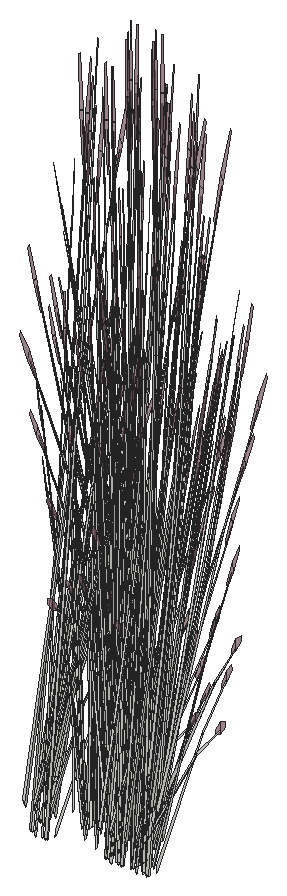
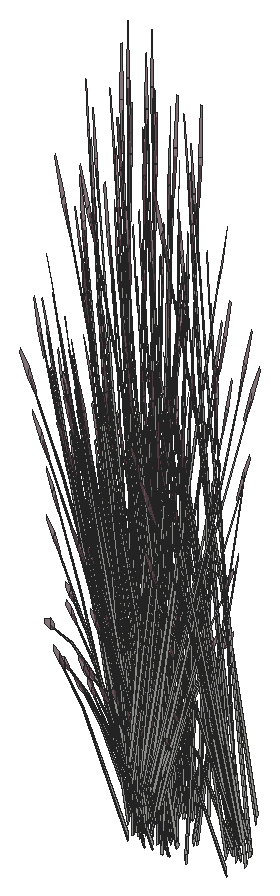
# SketchUp Ruby script. Lengths in inches.
U = 1.inch
M = Sketchup.active_model
def pt(a) = Geom::Point3d.new(a.map { |v| v * U })
def face(e, loops, mat)
  f = e.add_face(loops[0].map { |a| pt(a) })
  loops[1..].each { |l| e.add_face(l.map { |a| pt(a) }).erase! }
  f.material = f.back_material = mat if mat
  f
end
# faces: each face lists its corners as indices into pts; further lists are holes
def faces(e, pts, list, mat = nil) = list.each { |f| face(e, (f[0].is_a?(Array) ? f : [f]).map { |l| l.map { |i| pts[i] } }, mat) }
# xy, xz, yz: faces in a plane at the given z, y or x. An outline is a flat list of corners, or four numbers for a rectangle; further outlines are holes
def ring(l) = l.size == 4 ? [[l[0], l[1]], [l[2], l[1]], [l[2], l[3]], [l[0], l[3]]] : l.each_slice(2).to_a
def flat(e, list, mat, &to3) = list.each { |f| face(e, (f[0].is_a?(Array) ? f : [f]).map { |l| ring(l).map { |u, v| to3.(u, v) } }, mat) }
def xy(e, z, list, mat = nil) = flat(e, list, mat) { |x, y| [x, y, z] }
def xz(e, y, list, mat = nil) = flat(e, list, mat) { |x, z| [x, y, z] }
def yz(e, x, list, mat = nil) = flat(e, list, mat) { |y, z| [x, y, z] }
def lines(e, pts, list) = list.each { |a, b| e.add_line(pt(pts[a]), pt(pts[b])) }
# prism: a flat outline (further loops are holes) pulled along v
def prism(e, loops, v, mat = nil)
  f = face(e, loops, mat); d = Geom::Vector3d.new(v.map { |x| x * U })
  f.pushpull(f.normal.samedirection?(d) ? d.length : -d.length)
end
def box(e, o, s, mat = nil) = prism(e, [[o, [o[0] + s[0], o[1], o[2]], [o[0] + s[0], o[1] + s[1], o[2]], [o[0], o[1] + s[1], o[2]]]], [0, 0, s[2]], mat)
def at(x, y, z, deg = 0) = Geom::Transformation.translation(pt([x, y, z])) * Geom::Transformation.rotation(ORIGIN, Z_AXIS, deg.degrees)
def axes(o, x, y, z) = Geom::Transformation.new([*x, 0, *y, 0, *z, 0, *pt(o).to_a, 1])
def part(name) = M.definitions.add(name)
# library, detail: a bought-in or finely detailed component or shape, given as its bounding box
def library(name, o, s) = part(name).tap { |d| box(d.entities, o, s) }
def detail(e, o, s) = box(e.add_group.entities, o, s)
def put(e, d, t, mat = nil) = e.add_instance(d, t).tap { |i| i.material = mat if mat }
def group(e, t, mat = nil) = e.add_group.tap { |g| g.transformation = t; g.material = mat if mat }.entities
root = M.entities
M.materials.add("LightPink_Translucent").color = [144, 107, 117]
M.materials["LightPink_Translucent"].alpha = 0.75
c1 = part("blade")
p = [[2.15,0.21,22],[0,0.17,0],[0.09,0.45,0],[2.18,0.31,22],[2.29,0.31,22],[0.38,0.45,0],
  [2.48,0.24,33],[2.49,0.24,33],[2.48,0.22,33]]
faces(c1.entities,p,[[0,1,2,3],[4,5,2,3],[6,3,4,7],[8,0,3,6]])
c2 = part("seeds")
p = [[0.3,-0.1,1.38],[-0.01,-0.03,1.59],[-0.01,-0.03,0.03],[0.14,-0.07,-0.07],[0.29,-0.03,3],[0.15,0.01,3.11]]
faces(c2.entities,p,[[0,1,2,3],[1,0,4,5]],"LightPink_Translucent")
c3 = part("blade with seeds")
put(c3.entities,c1,at(0,0,0))
put(c3.entities,c2,axes([2.4,0.25,30.99],[1.5799,-0.05474,1.17369],[-0.12525,1.92788,0.29478],[-0.07173,-0.02425,1.56792]))
put(root,c3,axes([361.61,660.92,628.08],[0.3879,0.02311,-0.13498],[-0.0106,0.43749,-0.74919],[-0.02694,0.1685,1.13838]))
put(root,c3,axes([360.375,663.42,620.59],[-0.085,-0.1147,1.43002],[0.1106,-0.37943,-0.30754],[0.17198,0.0514,0.61141]))
put(root,c3,axes([362.33,661.41,627.71],[0.34538,-0.21713,-0.1216],[0.16972,0.38536,-0.67495],[0.04557,0.16239,1.02557]))
put(root,c3,axes([362.43,661.56,627.74],[-0.34777,-0.12192,0.53283],[0.11892,-0.40083,0.43934],[0.0209,0.15763,1.10256]))
put(root,c3,axes([361.79,662.16,625.45],[-0.00913,-0.2773,1.1486],[0.22824,0.19778,0.84392],[-0.04489,0.13217,0.25299]))
put(root,c3,axes([356.73,663.82,620.2],[0.35581,0.20937,0],[-0.17124,0.43505,0],[0,0,1.74954]))
put(root,c3,axes([358.86,663.83,620.2],[0.35581,0.20937,0],[-0.17124,0.43505,0],[0,0,1.74954]))
put(root,c3,axes([362.39,661.5,624.17],[0.05712,-0.02538,1.76342],[0.34359,0.13968,-0.26939],[0.01005,0.15742,0.30037]))
put(root,c3,axes([351.3,663.33,622.98],[0.35281,0.01123,-0.71045],[-0.0237,0.47284,0.08574],[0.14947,0.0499,1.00501]))
put(root,c3,axes([357.76,663.58,622.72],[0.07571,-0.00789,1.74944],[0.20767,-0.36231,-0.27667],[0.13467,0.04783,0.14031]))
put(root,c3,axes([356.87,664.28,620.19],[-0.21791,-0.46895,-0.05142],[0.36918,-0.26061,0.51607],[-0.09097,0.04465,1.6363]))
put(root,c3,axes([359.89,663.59,622.72],[0.07571,-0.00789,1.74944],[0.20767,-0.36231,-0.27667],[0.13467,0.04783,0.14031]))
put(root,c3,axes([359,664.3,620.19],[-0.21791,-0.46895,-0.05142],[0.36918,-0.26061,0.51607],[-0.09097,0.04465,1.6363]))
put(root,c3,axes([356.79,663.15,620.62],[0.26075,0.2802,0.1448],[-0.2175,0.31612,-0.41347],[-0.06054,0.04274,1.26744]))
put(root,c3,axes([358.92,663.16,620.62],[0.26075,0.2802,0.1448],[-0.2175,0.31612,-0.41347],[-0.06054,0.04274,1.26744]))
put(root,c3,axes([354.73,663.22,622.73],[-0.08753,-0.42921,0.48003],[0.34336,-0.07449,0.3958],[-0.1012,0.10094,0.9933]))
put(root,c3,axes([356.86,663.24,622.73],[-0.08753,-0.42921,0.48003],[0.34336,-0.07449,0.3958],[-0.1012,0.10094,0.9933]))
put(root,c3,axes([354.67,663.14,622.73],[-0.2423,-0.19613,0.0643],[0.14107,-0.2793,0.50621],[-0.07768,0.0903,0.77189]))
put(root,c3,axes([354.78,662.62,621.875],[0.12246,-0.09864,1.71376],[0.1031,0.45582,0.13857],[-0.19225,0.10302,0.73262]))
put(root,c3,axes([356.79,663.15,622.73],[-0.2423,-0.19613,0.0643],[0.14107,-0.2793,0.50621],[-0.07768,0.0903,0.77189]))
put(root,c3,axes([356.9,662.64,621.875],[0.12246,-0.09864,1.71376],[0.1031,0.45582,0.13857],[-0.19225,0.10302,0.73262]))
put(root,c3,axes([361.875,661.09,627.6875],[0.25266,0.31335,-0.5672],[-0.2669,0.27442,-0.43934],[-0.03844,0.15921,1.08528]))
put(root,c3,axes([361.6,661.56,625.5],[0.32063,-0.08258,0.06507],[0.07371,0.33271,-0.86304],[-0.02033,0.16842,0.7736]))
put(root,c3,axes([362.62,661.39,627.36],[0.34695,0.11691,-0.51099],[-0.11892,0.40083,-0.3958],[0.03181,0.16138,0.97773]))
put(root,c3,axes([362.82,660.57,626.56],[-0.08068,-0.14973,1.71376],[0.3728,-0.12606,0.13857],[0.08426,0.23506,0.73262]))
put(root,c3,axes([351.88,662.37,620.375],[0.44133,0,0],[0,0.52122,-0.51607],[0,0.11871,1.63711]))
put(root,c3,axes([357.47,663.63,622.98],[0.35281,0.01123,-0.71045],[-0.0237,0.47284,0.08574],[0.14947,0.0499,1.00501]))
put(root,c3,axes([359.6,663.65,622.98],[0.35281,0.01123,-0.71045],[-0.0237,0.47284,0.08574],[0.14947,0.0499,1.00501]))
put(root,c3,axes([350.75,662.1875,620.67],[0.39748,0.22252,-0.29095],[-0.19139,0.46966,-0.50002],[0.01249,0.11531,1.59708]))
put(root,c3,axes([357.07,664.01,620.48],[0.33032,-0.23318,0.49651],[0.19744,0.41812,0],[-0.07523,0.05311,1.57504]))
put(root,c3,axes([359.2,664.03,620.48],[0.33032,-0.23318,0.49651],[0.19744,0.41812,0],[-0.07523,0.05311,1.57504]))
put(root,c3,axes([362.46,661.64,627.21],[-0.1064,0.35863,-0.35414],[-0.31043,-0.1046,0.4572],[0.02846,0.14439,0.87481]))
put(root,c3,axes([351.51,663.53,622.53],[0.20082,0.29199,-0.35414],[-0.2293,0.2764,0.4572],[0.1165,0.04206,0.87481]))
put(root,c3,axes([351.61,662.72,620.03],[-0.24637,0.29097,-0.30978],[-0.24637,-0.29097,0.30978],[0,0.09372,1.38974]))
put(root,c3,axes([356.6,663.64,620.29],[0.15345,0.53576,-0.06012],[-0.43845,0.18773,0],[0.00536,0.01871,1.72173]))
put(root,c3,axes([358.73,663.66,620.29],[0.15345,0.53576,-0.06012],[-0.43845,0.18773,0],[0.00536,0.01871,1.72173]))
put(root,c3,axes([351.41,663.64,622.73],[-0.01777,0.35463,0.0643],[-0.26836,-0.00972,0.50621],[0.1028,0.03711,0.77189]))
put(root,c3,axes([356.77,664.22,620.03],[-0.32928,-0.11539,-0.30978],[0.08291,-0.40636,0.30978],[-0.06638,0.04686,1.38974]))
put(root,c3,axes([358.9,664.24,620.03],[-0.32928,-0.11539,-0.30978],[0.08291,-0.40636,0.30978],[-0.06638,0.04686,1.38974]))
put(root,c3,axes([354.39,663.4,620.59],[0.12266,0.03828,1.43002],[0.07906,0.39104,-0.30754],[-0.16661,0.0732,0.61141]))
put(root,c3,axes([361.8,660.95,628.02],[-0.00918,0.43138,-0.7886],[-0.38672,-0.02897,0.09517],[-0.04081,0.18275,1.11556]))
put(root,c3,axes([356.52,663.41,620.59],[0.12266,0.03828,1.43002],[0.07906,0.39104,-0.30754],[-0.16661,0.0732,0.61141]))
put(root,c3,axes([360.78,662.08,627.39],[0.04004,-0.02816,1.77383],[0.33095,0.18728,-0.16761],[-0.00778,0.15594,0.31391]))
put(root,c3,axes([354.94,663.08,623.05],[0.30722,-0.06665,0.35414],[0.08112,0.381,-0.4572],[-0.08804,0.10234,0.87481]))
put(root,c3,axes([351.43,663.53,622.73],[-0.26024,0.30729,0.48003],[-0.22444,-0.32634,0.3958],[0.1221,0.05668,0.9933]))
put(root,c3,axes([357.07,663.09,623.05],[0.30722,-0.06665,0.35414],[0.08112,0.381,-0.4572],[-0.08804,0.10234,0.87481]))
put(root,c3,axes([358.04,662.67,620.375],[0.44133,0,0],[0,0.52122,-0.51607],[0,0.11871,1.63711]))
put(root,c3,axes([360.17,662.6875,620.375],[0.44133,0,0],[0,0.52122,-0.51607],[0,0.11871,1.63711]))
put(root,c3,axes([353.76,662.91,622.71],[0.04504,0.01251,1.77383],[0.13934,0.41205,-0.16761],[-0.0922,0.10815,0.31391]))
put(root,c3,axes([357.87,662.94,620.2],[-0.44111,-0.00373,-0.04976],[0,-0.52122,0.49943],[-0.01386,0.11865,1.58352]))
put(root,c3,axes([355.89,662.92,622.71],[0.04504,0.01251,1.77383],[0.13934,0.41205,-0.16761],[-0.0922,0.10815,0.31391]))
put(root,c3,axes([360,662.96,620.2],[-0.44111,-0.00373,-0.04976],[0,-0.52122,0.49943],[-0.01386,0.11865,1.58352]))
put(root,c3,axes([356.91,662.49,620.67],[0.39748,0.22252,-0.29095],[-0.19139,0.46966,-0.50002],[0.01249,0.11531,1.59708]))
put(root,c3,axes([359.04,662.5,620.67],[0.39748,0.22252,-0.29095],[-0.19139,0.46966,-0.50002],[0.01249,0.11531,1.59708]))
put(root,c3,axes([362.16,660.64,626.56],[-0.00864,-0.17899,1.71376],[0.37441,0.11874,0.13857],[-0.02316,0.25508,0.73262]))
put(root,c3,axes([354.14,664.22,620.77],[0.14709,-0.21136,1.1486],[0.05804,0.3346,0.84392],[-0.1063,0.05991,0.25299]))
put(root,c3,axes([357.68,663.83,622.53],[0.20082,0.29199,-0.35414],[-0.2293,0.2764,0.4572],[0.1165,0.04206,0.87481]))
put(root,c3,axes([357.78,663.02,620.03],[-0.24637,0.29097,-0.30978],[-0.24637,-0.29097,0.30978],[0,0.09372,1.38974]))
put(root,c3,axes([356.27,664.23,620.77],[0.14709,-0.21136,1.1486],[0.05804,0.3346,0.84392],[-0.1063,0.05991,0.25299]))
put(root,c3,axes([359.81,663.84,622.53],[0.20082,0.29199,-0.35414],[-0.2293,0.2764,0.4572],[0.1165,0.04206,0.87481]))
put(root,c3,axes([359.9,663.03,620.03],[-0.24637,0.29097,-0.30978],[-0.24637,-0.29097,0.30978],[0,0.09372,1.38974]))
put(root,c3,axes([356.71,663.04,620.67],[0.04113,0.53214,-0.29095],[-0.42835,0.03218,-0.50002],[-0.07543,0.07088,1.59708]))
put(root,c3,axes([358.84,663.06,620.67],[0.04113,0.53214,-0.29095],[-0.42835,0.03218,-0.50002],[-0.07543,0.07088,1.59708]))
put(root,c3,axes([357.58,663.9375,622.73],[-0.01777,0.35463,0.0643],[-0.26836,-0.00972,0.50621],[0.1028,0.03711,0.77189]))
put(root,c3,axes([359.7,663.95,622.73],[-0.01777,0.35463,0.0643],[-0.26836,-0.00972,0.50621],[0.1028,0.03711,0.77189]))
put(root,c3,axes([356.87,662.84,620.21],[-0.17124,0.42022,-0.44739],[-0.35581,-0.20224,0.21531],[0,0.09687,1.43643]))
put(root,c3,axes([359,662.85,620.21],[-0.17124,0.42022,-0.44739],[-0.35581,-0.20224,0.21531],[0,0.09687,1.43643]))
put(root,c3,axes([354.69,663.3,622.53],[-0.30722,0.06665,-0.35414],[-0.08112,-0.381,0.4572],[-0.08804,0.10234,0.87481]))
put(root,c3,axes([356.82,663.32,622.53],[-0.30722,0.06665,-0.35414],[-0.08112,-0.381,0.4572],[-0.08804,0.10234,0.87481]))
put(root,c3,axes([362.5,661.32,627.66],[0.16845,0.3792,-0.71045],[-0.34676,0.21133,0.08574],[0.03939,0.18322,1.00501]))
put(root,c3,axes([357.6,663.83,622.73],[-0.26024,0.30729,0.48003],[-0.22444,-0.32634,0.3958],[0.1221,0.05668,0.9933]))
put(root,c3,axes([359.73,663.84,622.73],[-0.26024,0.30729,0.48003],[-0.22444,-0.32634,0.3958],[0.1221,0.05668,0.9933]))
put(root,c3,axes([350.61,663.88,623.05],[-0.05451,-0.37564,0.35414],[0.31161,-0.09919,-0.4572],[0.0837,0.10765,0.87481]))
put(root,c3,axes([351.78,662.73,620.02],[0,0.46636,-0.49651],[-0.39487,0,0],[0,0.10622,1.57504]))
put(root,c3,axes([361.52,661.91,625.27],[0.11138,-0.07357,1.43002],[0.27499,0.22183,-0.30754],[-0.08185,0.19194,0.61141]))
put(root,c3,axes([350.79,662.78,621.875],[-0.1311,-0.08035,1.71376],[0.27131,-0.33708,0.13857],[0.16909,0.15206,0.73262]))
put(root,c3,axes([362.24,662.27,627.4],[0.04474,0.0751,1.74944],[0.36104,0.0295,-0.27667],[0.03631,0.16562,0.14031]))
put(root,c3,axes([350.82,661.72,622.47],[-0.30498,-0.24231,1.38283],[0.32203,-0.37727,0.59665],[0.0984,0.22736,1.33663]))
put(root,c3,axes([354.25,664.16,623.65],[0.31145,0.12449,-0.06488],[-0.0958,0.38314,-0.29416],[-0.05094,0.05817,0.97024]))
put(root,c3,axes([356.46,663.45,620.06],[-0.23773,0.35053,-0.62353],[-0.29532,-0.31785,-0.16365],[-0.09526,0.08744,1.37633]))
put(root,c3,axes([356.375,664.18,623.65],[0.31145,0.12449,-0.06488],[-0.0958,0.38314,-0.29416],[-0.05094,0.05817,0.97024]))
put(root,c3,axes([358.58,663.47,620.06],[-0.23773,0.35053,-0.62353],[-0.29532,-0.31785,-0.16365],[-0.09526,0.08744,1.37633]))
put(root,c3,axes([351.28,663.69,620.77],[-0.19872,-0.13409,1.1486],[0.2566,-0.13625,0.84392],[0.06921,0.11541,0.25299]))
put(root,c3,axes([356.77,664.18,623.05],[-0.05451,-0.37564,0.35414],[0.31161,-0.09919,-0.4572],[0.0837,0.10765,0.87481]))
put(root,c3,axes([358.9,664.2,623.05],[-0.05451,-0.37564,0.35414],[0.31161,-0.09919,-0.4572],[0.0837,0.10765,0.87481]))
put(root,c3,axes([350.58,664.08,623.03],[0.21031,-0.39918,-0.1216],[0.30457,0.22997,-0.67495],[0.10587,0.11278,1.02557]))
put(root,c3,axes([356.88,664.04,620.33],[0.44186,0.15158,0.30756],[-0.11054,0.54181,-0.36492],[-0.07313,0.06781,1.64885]))
put(root,c3,axes([359.01,664.06,620.33],[0.44186,0.15158,0.30756],[-0.11054,0.54181,-0.36492],[-0.07313,0.06781,1.64885]))
put(root,c3,axes([356.85,664.41,620.02],[-0.33032,0.23318,-0.49651],[-0.19744,-0.41812,0],[-0.07523,0.05311,1.57504]))
put(root,c3,axes([357.94,663.03,620.02],[0,0.46636,-0.49651],[-0.39487,0,0],[0,0.10622,1.57504]))
put(root,c3,axes([358.98,664.42,620.02],[-0.33032,0.23318,-0.49651],[-0.19744,-0.41812,0],[-0.07523,0.05311,1.57504]))
put(root,c3,axes([360.07,663.04,620.02],[0,0.46636,-0.49651],[-0.39487,0,0],[0,0.10622,1.57504]))
put(root,c3,axes([356.96,663.08,621.875],[-0.1311,-0.08035,1.71376],[0.27131,-0.33708,0.13857],[0.16909,0.15206,0.73262]))
put(root,c3,axes([359.09,663.09,621.875],[-0.1311,-0.08035,1.71376],[0.27131,-0.33708,0.13857],[0.16909,0.15206,0.73262]))
put(root,c3,axes([356.98,662.02,622.47],[-0.30498,-0.24231,1.38283],[0.32203,-0.37727,0.59665],[0.0984,0.22736,1.33663]))
put(root,c3,axes([359.11,662.04,622.47],[-0.30498,-0.24231,1.38283],[0.32203,-0.37727,0.59665],[0.0984,0.22736,1.33663]))
put(root,c3,axes([354.79,663.04,623.03],[0.32648,0.25715,-0.1216],[-0.18809,0.3724,-0.67495],[-0.09224,0.12945,1.02557]))
put(root,c3,axes([356.91,663.06,623.03],[0.32648,0.25715,-0.1216],[-0.18809,0.3724,-0.67495],[-0.09224,0.12945,1.02557]))
put(root,c3,axes([353.23,669.87,627.46],[0.08068,0.14973,1.71376],[-0.3728,0.12606,0.13857],[-0.08426,-0.23506,0.73262]))
put(root,c3,axes([357.44,663.99,620.77],[-0.19872,-0.13409,1.1486],[0.2566,-0.13625,0.84392],[0.06921,0.11541,0.25299]))
put(root,c3,axes([359.57,664.01,620.77],[-0.19872,-0.13409,1.1486],[0.2566,-0.13625,0.84392],[0.06921,0.11541,0.25299]))
put(root,c3,axes([361.67,661.55,626.04],[0.00775,-0.24075,1.54345],[0.34877,0.12716,0.21329],[-0.03022,0.25658,0.72882]))
put(root,c3,axes([350.3,664.41,622.71],[0.00104,-0.05646,1.77383],[0.30246,-0.2491,-0.16761],[0.10506,0.08891,0.31391]))
put(root,c3,axes([356.75,664.375,623.03],[0.21031,-0.39918,-0.1216],[0.30457,0.22997,-0.67495],[0.10587,0.11278,1.02557]))
put(root,c3,axes([358.875,664.39,623.03],[0.21031,-0.39918,-0.1216],[0.30457,0.22997,-0.67495],[0.10587,0.11278,1.02557]))
put(root,c3,axes([351.33,664.19,619.49],[0.02571,-0.06733,1.76342],[0.32373,-0.19829,-0.26939],[0.09815,0.10263,0.30037]))
put(root,c3,axes([350.91,662.66,620.09],[0.12941,0.42699,-0.69212],[-0.37279,0.15378,-0.18165],[0.0143,0.14459,1.52773]))
put(root,c3,axes([353.85,668.88,628.3],[-0.05398,-0.06539,1.74944],[-0.36026,0.04145,-0.27667],[-0.0575,-0.15639,0.14031]))
put(root,c3,axes([350.83,663.88,622.68],[0.34827,-0.11086,-0.51099],[0.06092,0.41983,-0.3958],[0.09354,0.12031,0.97773]))
put(root,c3,axes([355.22,662.93,621.875],[0.08815,-0.14329,1.71376],[0.22258,0.38678,0.13857],[-0.15267,0.17614,0.73262]))
put(root,c3,axes([357.35,662.94,621.875],[0.08815,-0.14329,1.71376],[0.22258,0.38678,0.13857],[-0.15267,0.17614,0.73262]))
put(root,c3,axes([354.68,669.65,626.18],[-0.10032,0.0944,1.43002],[-0.30046,-0.16522,-0.30754],[0.05569,-0.20547,0.61141]))
put(root,c3,axes([354.95,663.35,622.68],[0.09067,0.42583,-0.51099],[-0.34336,0.07449,-0.3958],[-0.0984,0.11438,0.97773]))
put(root,c3,axes([357.08,663.36,622.68],[0.09067,0.42583,-0.51099],[-0.34336,0.07449,-0.3958],[-0.0984,0.11438,0.97773]))
put(root,c3,axes([354.22,669.98,628.57],[-0.16845,-0.3792,-0.71045],[0.34676,-0.21133,0.08574],[-0.03939,-0.18322,1.00501]))
put(root,c3,axes([355.36,663.84,623.05],[0.23881,-0.24554,0.35414],[0.22606,0.28036,-0.4572],[-0.0344,0.14245,0.87481]))
put(root,c3,axes([357.49,663.85,623.05],[0.23881,-0.24554,0.35414],[0.22606,0.28036,-0.4572],[-0.0344,0.14245,0.87481]))
put(root,c3,axes([357.15,664.33,620.375],[0.22066,0.46731,0],[-0.36918,0.26061,-0.51607],[-0.08408,0.05936,1.63711]))
put(root,c3,axes([353.13,669.48,626.18],[-0.02137,0.15256,1.43002],[-0.31245,0.12771,-0.30754],[-0.07303,-0.19719,0.61141]))
put(root,c3,axes([359.28,664.35,620.375],[0.22066,0.46731,0],[-0.36918,0.26061,-0.51607],[-0.08408,0.05936,1.63711]))
put(root,c3,axes([356.47,664.71,622.71],[0.00104,-0.05646,1.77383],[0.30246,-0.2491,-0.16761],[0.10506,0.08891,0.31391]))
put(root,c3,axes([358.6,664.72,622.71],[0.00104,-0.05646,1.77383],[0.30246,-0.2491,-0.16761],[0.10506,0.08891,0.31391]))
put(root,c3,axes([357.5,664.49,619.49],[0.02571,-0.06733,1.76342],[0.32373,-0.19829,-0.26939],[0.09815,0.10263,0.30037]))
put(root,c3,axes([351.31,664.3,620.67],[-0.22633,-0.01463,1.0506],[0.14947,-0.31064,0.58006],[0.08941,0.11036,0.8241]))
put(root,c3,axes([356.96,662.48,620.84],[-0.00964,-0.43909,1.41272],[0.43635,0.11382,0.59816],[-0.1032,0.24027,1.3335]))
put(root,c3,axes([359.63,664.51,619.49],[0.02571,-0.06733,1.76342],[0.32373,-0.19829,-0.26939],[0.09815,0.10263,0.30037]))
put(root,c3,axes([357.07,662.96,620.09],[0.12941,0.42699,-0.69212],[-0.37279,0.15378,-0.18165],[0.0143,0.14459,1.52773]))
put(root,c3,axes([355.14,664.06,622.73],[-0.29004,-0.02173,0.0643],[0.00795,-0.32812,0.50621],[-0.03035,0.12569,0.77189]))
put(root,c3,axes([359.09,662.5,620.84],[-0.00964,-0.43909,1.41272],[0.43635,0.11382,0.59816],[-0.1032,0.24027,1.3335]))
put(root,c3,axes([359.2,662.98,620.09],[0.12941,0.42699,-0.69212],[-0.37279,0.15378,-0.18165],[0.0143,0.14459,1.52773]))
put(root,c3,axes([357.27,664.08,622.73],[-0.29004,-0.02173,0.0643],[0.00795,-0.32812,0.50621],[-0.03035,0.12569,0.77189]))
put(root,c3,axes([354.53,664.43,619.49],[0.04734,0.04659,1.76342],[0.08027,0.4317,-0.26939],[-0.10492,0.09206,0.30037]))
put(root,c3,axes([353.93,669.14,625.08],[-0.0592,0.0168,1.76342],[-0.32738,-0.18913,-0.26939],[0.00549,-0.15776,0.30037]))
put(root,c3,axes([356.65,664.45,619.49],[0.04734,0.04659,1.76342],[0.08027,0.4317,-0.26939],[-0.10492,0.09206,0.30037]))
put(root,c3,axes([355.23,664.09,622.73],[-0.25132,-0.3182,0.48003],[0.2669,-0.27442,0.3958],[-0.04636,0.14929,0.9933]))
put(root,c3,axes([356.99,664.18,622.68],[0.34827,-0.11086,-0.51099],[0.06092,0.41983,-0.3958],[0.09354,0.12031,0.97773]))
put(root,c3,axes([357.36,664.11,622.73],[-0.25132,-0.3182,0.48003],[0.2669,-0.27442,0.3958],[-0.04636,0.14929,0.9933]))
put(root,c3,axes([359.12,664.19,622.68],[0.34827,-0.11086,-0.51099],[0.06092,0.41983,-0.3958],[0.09354,0.12031,0.97773]))
put(root,c3,axes([350.66,664.22,622.73],[-0.16041,0.29625,0.0643],[-0.22843,-0.17248,0.50621],[0.07385,0.09498,0.77189]))
put(root,c3,axes([356.03,664.24,623.05],[0.1064,-0.35863,0.35414],[0.31043,0.1046,-0.4572],[0.02846,0.14439,0.87481]))
put(root,c3,axes([358.16,664.26,623.05],[0.1064,-0.35863,0.35414],[0.31043,0.1046,-0.4572],[0.02846,0.14439,0.87481]))
put(root,c3,axes([354.93,670.35,628.57],[0.00918,-0.43138,-0.71045],[0.38672,0.02897,0.08574],[0.04081,-0.18275,1.00501]))
put(root,c3,axes([350.72,664.14,622.73],[-0.35104,0.10702,0.48003],[-0.06092,-0.41983,0.3958],[0.08256,0.12373,0.9933]))
put(root,c3,axes([357.48,664.6,620.67],[-0.22633,-0.01463,1.0506],[0.14947,-0.31064,0.58006],[0.08941,0.11036,0.8241]))
put(root,c3,axes([359.6,664.62,620.67],[-0.22633,-0.01463,1.0506],[0.14947,-0.31064,0.58006],[0.08941,0.11036,0.8241]))
put(root,c3,axes([355.46,669.68,628.3],[-0.00341,-0.09282,1.74944],[-0.28775,-0.26825,-0.27667],[0.04449,-0.16261,0.14031]))
put(root,c3,axes([354.26,669.66,628.12],[0.1064,-0.35863,-0.35414],[0.31043,0.1046,0.4572],[-0.02846,-0.14439,0.87481]))
put(root,c3,axes([354.49,670.13,627.46],[-0.06572,0.16029,1.71376],[-0.27569,-0.33172,0.13857],[0.12437,-0.20675,0.73262]))
put(root,c3,axes([355.39,669.35,628.3],[-0.03584,0.03562,1.77383],[-0.35118,-0.12018,-0.16761],[-0.01271,-0.15545,0.31391]))
put(root,c3,axes([356.82,664.52,622.73],[-0.16041,0.29625,0.0643],[-0.22843,-0.17248,0.50621],[0.07385,0.09498,0.77189]))
put(root,c3,axes([350.57,663.55,620.59],[0.00623,-0.15459,1.43002],[0.29764,-0.17268,-0.30754],[0.09188,0.18503,0.61141]))
put(root,c3,axes([358.95,664.54,622.73],[-0.16041,0.29625,0.0643],[-0.22843,-0.17248,0.50621],[0.07385,0.09498,0.77189]))
put(root,c3,axes([356.45,665.52,623.65],[0.2439,-0.26754,-0.06488],[0.22348,0.29302,-0.29416],[0.01573,0.08303,0.97024]))
put(root,c3,axes([358.57,665.54,623.65],[0.2439,-0.26754,-0.06488],[0.22348,0.29302,-0.29416],[0.01573,0.08303,0.97024]))
put(root,c3,axes([354.1,669.91,628.27],[-0.34695,-0.11691,-0.51099],[0.11892,-0.40083,-0.3958],[-0.03181,-0.16138,0.97773]))
put(root,c3,axes([354.3125,668.9,626.35],[0.04528,0.27194,1.1486],[-0.25117,-0.15062,0.84392],[0.02703,-0.13924,0.25299]))
put(root,c3,axes([356.89,664.4375,622.73],[-0.35104,0.10702,0.48003],[-0.06092,-0.41983,0.3958],[0.08256,0.12373,0.9933]))
put(root,c3,axes([359.02,664.45,622.73],[-0.35104,0.10702,0.48003],[-0.06092,-0.41983,0.3958],[0.08256,0.12373,0.9933]))
put(root,c3,axes([349.76,664.09,623.03],[0.34538,-0.21713,-0.1216],[0.16972,0.38536,-0.67495],[0.04557,0.16239,1.02557]))
put(root,c3,axes([354.85,670.21,628.27],[-0.25266,-0.31335,-0.51099],[0.2669,-0.27442,-0.3958],[0.03844,-0.15921,0.97773]))
put(root,c3,axes([355.16,663.28,621.875],[0.06572,-0.16029,1.71376],[0.27569,0.33172,0.13857],[-0.12437,0.20675,0.73262]))
put(root,c3,axes([357.29,663.3,621.875],[0.06572,-0.16029,1.71376],[0.27569,0.33172,0.13857],[-0.12437,0.20675,0.73262]))
put(root,c3,axes([353.48,668.66,628.3],[-0.00658,0.0559,1.77383],[-0.32474,0.20287,-0.16761],[-0.09556,-0.1037,0.31391]))
put(root,c3,axes([356.74,663.85,620.59],[0.00623,-0.15459,1.43002],[0.29764,-0.17268,-0.30754],[0.09188,0.18503,0.61141]))
put(root,c3,axes([358.86,663.87,620.59],[0.00623,-0.15459,1.43002],[0.29764,-0.17268,-0.30754],[0.09188,0.18503,0.61141]))
put(root,c3,axes([355.93,664.57,622.73],[-0.26007,0.1585,0.0643],[-0.12729,-0.28902,0.50621],[0.02512,0.1274,0.77189]))
put(root,c3,axes([358.06,664.58,622.73],[-0.26007,0.1585,0.0643],[-0.12729,-0.28902,0.50621],[0.02512,0.1274,0.77189]))
put(root,c3,axes([355.23,664.1875,622.53],[-0.23881,0.24554,-0.35414],[-0.22606,-0.28036,0.4572],[-0.0344,0.14245,0.87481]))
put(root,c3,axes([354.41,664.11,622.72],[-0.00877,0.09229,1.74944],[0.24897,0.32105,-0.27667],[-0.06518,0.15182,0.14031]))
put(root,c3,axes([353.4,669.66,628.68],[0.39316,-0.11987,0.53763],[0.06823,0.47021,0.4433],[-0.09247,-0.13858,1.11249]))
put(root,c3,axes([357.36,664.2,622.53],[-0.23881,0.24554,-0.35414],[-0.22606,-0.28036,0.4572],[-0.0344,0.14245,0.87481]))
put(root,c3,axes([356.54,664.13,622.72],[-0.00877,0.09229,1.74944],[0.24897,0.32105,-0.27667],[-0.06518,0.15182,0.14031]))
put(root,c3,axes([355.21,663.9,623.4],[0.3879,0.02311,-0.13498],[-0.0106,0.43749,-0.74919],[-0.02694,0.1685,1.13838]))
put(root,c3,axes([357.34,663.92,623.4],[0.3879,0.02311,-0.13498],[-0.0106,0.43749,-0.74919],[-0.02694,0.1685,1.13838]))
put(root,c3,axes([355.92,664.39,623.03],[0.34538,-0.21713,-0.1216],[0.16972,0.38536,-0.67495],[0.04557,0.16239,1.02557]))
put(root,c3,axes([358.05,664.41,623.03],[0.34538,-0.21713,-0.1216],[0.16972,0.38536,-0.67495],[0.04557,0.16239,1.02557]))
put(root,c3,axes([356.02,664.54,623.0625],[-0.34777,-0.12192,0.53283],[0.11892,-0.40083,0.43934],[0.0209,0.15763,1.10256]))
put(root,c3,axes([358.15,664.55,623.0625],[-0.34777,-0.12192,0.53283],[0.11892,-0.40083,0.43934],[0.0209,0.15763,1.10256]))
put(root,c3,axes([354.29,669.74,628.32],[0.34777,0.12192,0.48003],[-0.11892,0.40083,0.3958],[-0.0209,-0.15763,0.9933]))
put(root,c3,axes([355.39,665.14,620.77],[-0.00913,-0.2773,1.1486],[0.22824,0.19778,0.84392],[-0.04489,0.13217,0.25299]))
put(root,c3,axes([354.39,669.89,628.62],[-0.34538,0.21713,-0.1216],[-0.16972,-0.38536,-0.67495],[-0.04557,-0.16239,1.02557]))
put(root,c3,axes([357.51,665.15,620.77],[-0.00913,-0.2773,1.1486],[0.22824,0.19778,0.84392],[-0.04489,0.13217,0.25299]))
put(root,c3,axes([355.11,670.375,628.62],[-0.3879,-0.02311,-0.1216],[0.0106,-0.43749,-0.67495],[0.02694,-0.1685,1.02557]))
put(root,c3,axes([355.08,670.09,628.12],[0.23881,-0.24554,-0.35414],[0.22606,0.28036,0.4572],[0.0344,-0.14245,0.87481]))
put(root,c3,axes([353.02,669.23,626.35],[0.18411,0.16231,1.1486],[-0.26813,0.09757,0.84392],[-0.05737,-0.12474,0.25299]))
put(root,c3,axes([354.39,669.71,628.32],[0.26007,-0.1585,0.0643],[0.12729,0.28902,0.50621],[-0.02512,-0.1274,0.77189]))
put(root,c3,axes([353.46,670.09,628.57],[-0.30095,-0.22541,-0.71045],[0.21388,-0.395,0.08574],[-0.10904,-0.13459,1.00501]))
put(root,c3,axes([350.05,664.07,622.68],[0.34695,0.11691,-0.51099],[-0.11892,0.40083,-0.3958],[0.03181,0.16138,0.97773]))
put(root,c3,axes([350.25,663.25,621.875],[-0.08068,-0.14973,1.71376],[0.3728,-0.12606,0.13857],[0.08426,0.23506,0.73262]))
put(root,c3,axes([353.36,669.79,628.12],[-0.05451,-0.37564,-0.35414],[0.31161,-0.09919,0.4572],[-0.0837,-0.10765,0.87481]))
put(root,c3,axes([355.99,664.48,619.49],[0.05712,-0.02538,1.76342],[0.34359,0.13968,-0.26939],[0.01005,0.15742,0.30037]))
put(root,c3,axes([358.12,664.49,619.49],[0.05712,-0.02538,1.76342],[0.34359,0.13968,-0.26939],[0.01005,0.15742,0.30037]))
put(root,c3,axes([355.47,664.07,623],[0.25266,0.31335,-0.5672],[-0.2669,0.27442,-0.43934],[-0.03844,0.15921,1.08528]))
put(root,c3,axes([357.6,664.08,623],[0.25266,0.31335,-0.5672],[-0.2669,0.27442,-0.43934],[-0.03844,0.15921,1.08528]))
put(root,c3,axes([355.2,664.54,620.82],[0.32063,-0.08258,0.06507],[0.07371,0.33271,-0.86304],[-0.02033,0.16842,0.7736]))
